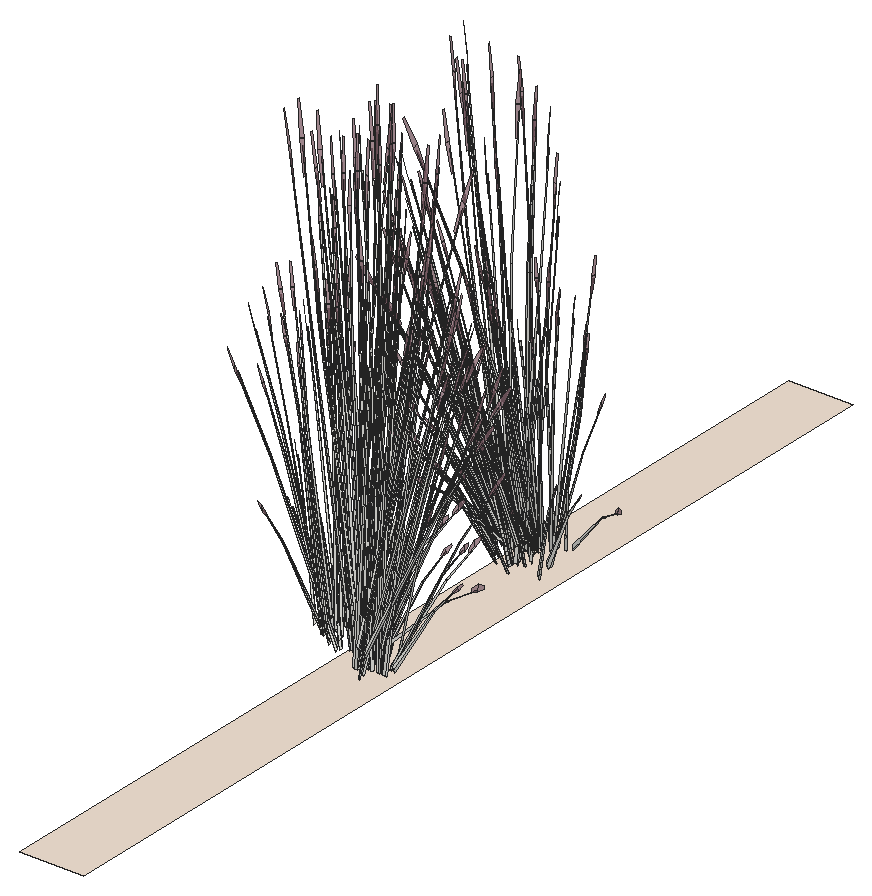
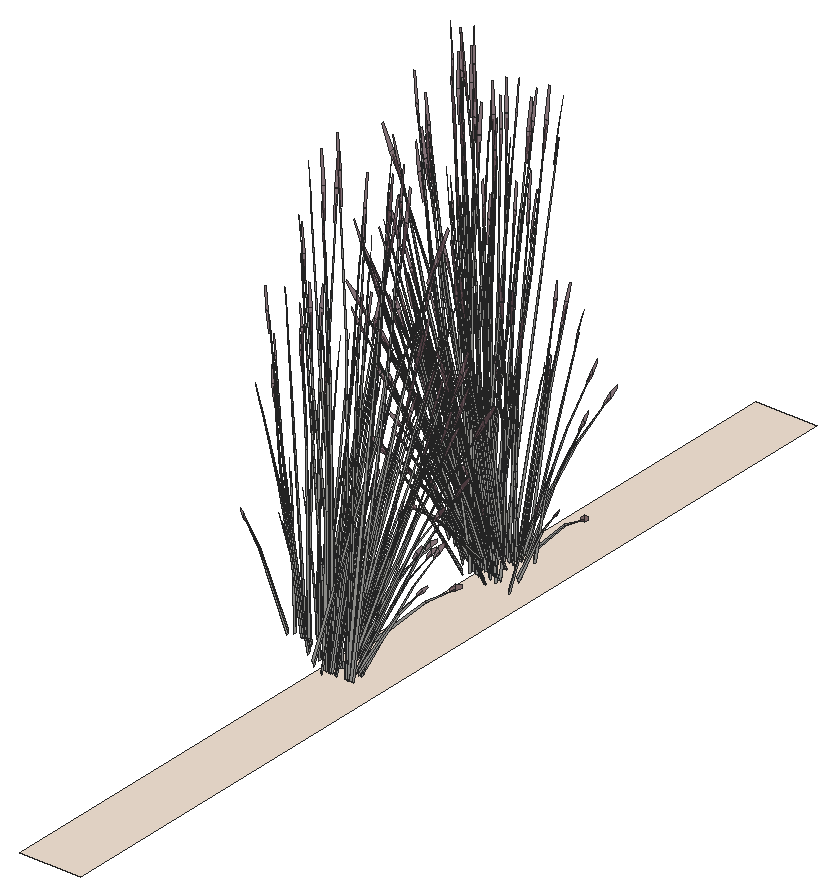
# SketchUp Ruby script. Lengths in inches.
U = 1.inch
M = Sketchup.active_model
def pt(a) = Geom::Point3d.new(a.map { |v| v * U })
def face(e, loops, mat)
  f = e.add_face(loops[0].map { |a| pt(a) })
  loops[1..].each { |l| e.add_face(l.map { |a| pt(a) }).erase! }
  f.material = f.back_material = mat if mat
  f
end
# faces: each face lists its corners as indices into pts; further lists are holes
def faces(e, pts, list, mat = nil) = list.each { |f| face(e, (f[0].is_a?(Array) ? f : [f]).map { |l| l.map { |i| pts[i] } }, mat) }
# xy, xz, yz: faces in a plane at the given z, y or x. An outline is a flat list of corners, or four numbers for a rectangle; further outlines are holes
def ring(l) = l.size == 4 ? [[l[0], l[1]], [l[2], l[1]], [l[2], l[3]], [l[0], l[3]]] : l.each_slice(2).to_a
def flat(e, list, mat, &to3) = list.each { |f| face(e, (f[0].is_a?(Array) ? f : [f]).map { |l| ring(l).map { |u, v| to3.(u, v) } }, mat) }
def xy(e, z, list, mat = nil) = flat(e, list, mat) { |x, y| [x, y, z] }
def xz(e, y, list, mat = nil) = flat(e, list, mat) { |x, z| [x, y, z] }
def yz(e, x, list, mat = nil) = flat(e, list, mat) { |y, z| [x, y, z] }
def lines(e, pts, list) = list.each { |a, b| e.add_line(pt(pts[a]), pt(pts[b])) }
# prism: a flat outline (further loops are holes) pulled along v
def prism(e, loops, v, mat = nil)
  f = face(e, loops, mat); d = Geom::Vector3d.new(v.map { |x| x * U })
  f.pushpull(f.normal.samedirection?(d) ? d.length : -d.length)
end
def box(e, o, s, mat = nil) = prism(e, [[o, [o[0] + s[0], o[1], o[2]], [o[0] + s[0], o[1] + s[1], o[2]], [o[0], o[1] + s[1], o[2]]]], [0, 0, s[2]], mat)
def at(x, y, z, deg = 0) = Geom::Transformation.translation(pt([x, y, z])) * Geom::Transformation.rotation(ORIGIN, Z_AXIS, deg.degrees)
def axes(o, x, y, z) = Geom::Transformation.new([*x, 0, *y, 0, *z, 0, *pt(o).to_a, 1])
def part(name) = M.definitions.add(name)
# library, detail: a bought-in or finely detailed component or shape, given as its bounding box
def library(name, o, s) = part(name).tap { |d| box(d.entities, o, s) }
def detail(e, o, s) = box(e.add_group.entities, o, s)
def put(e, d, t, mat = nil) = e.add_instance(d, t).tap { |i| i.material = mat if mat }
def group(e, t, mat = nil) = e.add_group.tap { |g| g.transformation = t; g.material = mat if mat }.entities
root = M.entities
M.materials.add("C01_Vanilla_Cream").color = [244, 228, 212]
M.materials.add("LightPink_Translucent").color = [144, 107, 117]
M.materials["LightPink_Translucent"].alpha = 0.75
c1 = part("blade")
p = [[2.15,0.21,22],[0,0.17,0],[0.09,0.45,0],[2.18,0.31,22],[2.29,0.31,22],[0.38,0.45,0],
  [2.48,0.24,33],[2.49,0.24,33],[2.48,0.22,33]]
faces(c1.entities,p,[[0,1,2,3],[4,5,2,3],[6,3,4,7],[8,0,3,6]])
c2 = part("seeds")
p = [[0.3,-0.1,1.38],[-0.01,-0.03,1.59],[-0.01,-0.03,0.03],[0.14,-0.07,-0.07],[0.29,-0.03,3],[0.15,0.01,3.11]]
faces(c2.entities,p,[[0,1,2,3],[1,0,4,5]],"LightPink_Translucent")
c3 = part("blade with seeds")
put(c3.entities,c1,at(0,0,0))
put(c3.entities,c2,axes([2.4,0.25,30.99],[1.5799,-0.05474,1.17369],[-0.12525,1.92788,0.29478],[-0.07173,-0.02425,1.56792]))
xy(root,48,[[354,216,360,306.76]],"C01_Vanilla_Cream")
put(root,c3,axes([358.93,250.65,50.91],[-0.23093,0.01116,1.28532],[0.15319,-0.4836,0.10393],[0.32909,0.02991,0.54946]))
put(root,c3,axes([359.23,249.6,49.52],[0.13078,0.42928,-0.23233],[-0.51941,0.1219,0.23233],[0.10471,0.0495,1.0423]))
put(root,c3,axes([360.13,251.32,51.55],[0.20448,0.33592,0.04823],[-0.37288,0.16442,0.37966],[0.16437,-0.03244,0.57892]))
put(root,c3,axes([358.1875,250.5625,49.79],[-0.70367,-0.1038,0.36899],[0.1432,-0.58624,0.1448],[0.10283,0.05661,1.2811]))
put(root,c3,axes([360.09,251.2,51.55],[-0.15729,0.44921,0.36002],[-0.51712,-0.15361,0.29685],[0.20336,-0.027,0.74497]))
put(root,c3,axes([357.625,252.01,49.65],[-0.18165,-0.42474,0],[0.51872,-0.14874,0],[0,0,1.15778]))
put(root,c3,axes([357.28,251.61,49.96],[-0.1074,0.43968,0.1086],[-0.52474,-0.07632,-0.3101],[-0.0955,-0.04515,0.95058]))
put(root,c3,axes([355.24,250.47,51.79],[0.46269,0.13744,0.2656],[-0.13495,0.40096,-0.3429],[-0.18628,0.03677,0.65611]))
put(root,c3,axes([358.31,251.95,49.64],[0.5845,-0.16716,-0.14398],[0.20539,0.48152,0.00006],[0.06452,-0.01848,1.30423]))
put(root,c3,axes([358.51,252.15,49.86],[0.16083,-0.48962,0.13232],[0.58854,0.13856,0.26315],[-0.10167,0.00238,1.20305]))
put(root,c3,axes([358.375,251.04,49.66],[0.38863,0.31822,0],[-0.38863,0.31822,0],[0,0,1.2695]))
put(root,c3,axes([356.17,250.44,50.51],[0.15825,-0.07127,1.32798],[0.05457,0.4976,0.10393],[-0.34278,0.06603,0.47463]))
put(root,c3,axes([359.43,250.9,49.86],[-0.43742,-0.35886,0.13232],[0.44081,-0.34807,0.26315],[-0.04831,0.07329,1.20305]))
put(root,c3,axes([358.62,250.36,49.54],[0.57914,0.08077,-0.46765],[-0.12221,0.49823,-0.12274],[0.17283,0.06037,1.03225]))
put(root,c3,axes([361.18,251.23,50.07],[-0.34399,0.08133,0.86145],[0.16192,-0.33614,0.63294],[0.18249,0.023,0.18974]))
put(root,c3,axes([357.5,252.2,49.65],[-0.56127,-0.22118,0],[0.27012,-0.45959,0],[0,0,1.2203]))
put(root,c3,axes([357.96,251.61,49.85],[-0.54364,-0.39653,-0.18894],[0.45745,-0.44527,0.41347],[-0.14639,0.04639,1.26162]))
put(root,c3,axes([356.53,252.375,49.86],[0.52105,0.24633,0.37238],[-0.31144,0.44171,0],[-0.11867,-0.0561,1.18128]))
put(root,c3,axes([358.37,250.67,50.04],[0.27012,-0.44393,0.33554],[0.56127,0.21365,-0.16149],[0,0.10233,1.07733]))
put(root,c3,axes([361.02,252.65,51.53],[-0.05034,-0.04313,1.33037],[0.11012,-0.46232,-0.12571],[0.1983,-0.02954,0.23543]))
put(root,c3,axes([354.47,250.78,51.54],[-0.09091,0.06396,1.31208],[0.00773,0.46734,-0.2075],[-0.20839,0.06078,0.10523]))
put(root,c3,axes([358.27,250.92,49.72],[0,0.56976,-0.04228],[-0.69617,0,0],[0,0.01791,1.34526]))
put(root,c3,axes([355.07,250.72,51.51],[-0.15083,0.44814,-0.38324],[-0.51712,-0.15361,-0.29685],[-0.2082,0.04109,0.7333]))
put(root,c3,axes([355.05,250.33,51.78],[0.28012,0.44611,-0.0912],[-0.49717,0.21923,-0.50621],[-0.20951,0.05886,0.76918]))
put(root,c3,axes([358.32,250.52,49.66],[0.33445,0.41351,-0.33554],[-0.50659,0.29119,0.16149],[0.10823,0.05117,1.07733]))
put(root,c3,axes([360.58,252.27,50.95],[-0.10656,-0.41414,-0.02619],[0.50364,-0.09521,-0.11874],[0.10517,0.02626,0.39164]))
put(root,c3,axes([356.23,252.63,49.78],[-0.34808,0.49367,0],[-0.58235,-0.27531,-0.38706],[-0.13264,-0.0627,1.22783]))
put(root,c3,axes([359.27,252.26,51.78],[0.02981,-0.50103,-0.0912],[0.56442,0.01369,-0.50621],[0.21738,0.0348,0.76918]))
put(root,c3,axes([359.79,250.92,49.86],[0,-0.49266,0.37238],[0.62289,0,0],[0,0.11221,1.18128]))
put(root,c3,axes([358.23,251.29,50.04],[0.60457,-0.03041,0.33554],[0.05467,0.50484,-0.16149],[-0.10823,0.05117,1.07733]))
put(root,c3,axes([358.6,250.77,49.96],[0.51872,-0.14368,0.1086],[0.18165,0.41027,-0.3101],[0,0.09029,0.95058]))
put(root,c3,axes([359.1875,252.06,51.79],[-0.31678,-0.30846,0.2656],[0.36171,-0.29199,-0.3429],[0.18378,0.04443,0.65611]))
put(root,c3,axes([357.6875,251.53,49.66],[-0.60457,0.03041,-0.33554],[-0.05467,-0.50484,0.16149],[-0.10823,0.05117,1.07733]))
put(root,c3,axes([360.53,251.77,49.94],[-0.13408,-0.12117,1.07251],[0.17446,-0.40083,-0.23066],[0.27128,0.0543,0.45856]))
put(root,c3,axes([358.14,252.21,49.65],[0.56127,0.22118,0],[-0.27012,0.45959,0],[0,0,1.31215]))
put(root,c3,axes([359.76,251.95,51.54],[0.11943,-0.00833,1.31208],[0.32759,-0.38275,-0.2075],[0.21244,0.05052,0.10523]))
put(root,c3,axes([358.36,252.7,49.64],[-0.34375,-0.4954,-0.03857],[0.58235,-0.27531,0.38706],[-0.1435,0.04717,1.22723]))
put(root,c3,axes([358.24,251.5,49.96],[0.41131,0.296,0.1086],[-0.34309,0.33395,-0.3101],[-0.0955,0.04515,0.95058]))
put(root,c3,axes([354.99,251.58,51.55],[-0.13808,-0.45342,0.36002],[0.54163,-0.07869,0.29685],[-0.15963,0.10664,0.74497]))
put(root,c3,axes([354.88,251.49,51.55],[-0.3822,-0.20719,0.04823],[0.22252,-0.29505,0.37966],[-0.12254,0.09539,0.57892]))
put(root,c3,axes([355.06,250.95,50.91],[0.19317,-0.10421,1.28532],[0.16263,0.48153,0.10393],[-0.30326,0.10883,0.54946]))
put(root,c3,axes([359.3,252.01,51.74],[0.55654,0.01186,-0.53284],[-0.03738,0.49951,0.0643],[0.23578,0.05271,0.75375]))
put(root,c3,axes([358.67,252.41,49.86],[0.52105,-0.24633,0.37238],[0.31144,0.44171,0],[-0.11867,0.0561,1.18128]))
put(root,c3,axes([357.93,252.03,49.72],[0.24206,0.56598,-0.04509],[-0.69162,0.19832,0],[0.00845,0.01976,1.2913]))
put(root,c3,axes([358.2,252.64,49.52],[-0.51941,-0.1219,-0.23233],[0.13078,-0.42928,0.23233],[-0.10471,0.0495,1.0423]))
put(root,c3,axes([354.45,251.77,49.94],[0.19348,0.04044,1.07251],[0.1247,0.41309,-0.23066],[-0.26282,0.07733,0.45856]))
put(root,c3,axes([355.32,251.43,51.79],[0.48462,-0.07041,0.2656],[0.12797,0.4025,-0.3429],[-0.13888,0.10811,0.65611]))
put(root,c3,axes([360.21,251,49.78],[0.69617,0,0],[0,0.55062,-0.38706],[0,0.12541,1.22783]))
put(root,c3,axes([353.46,251.25,51.53],[0.07105,0.01321,1.33037],[0.2198,0.43529,-0.12571],[-0.14545,0.11425,0.23543]))
put(root,c3,axes([359.93,251.28,49.65],[-0.69582,-0.00394,-0.03732],[0,-0.55062,0.37457],[-0.02187,0.12535,1.18764]))
put(root,c3,axes([358.43,250.8,50],[0.62699,0.23507,-0.21822],[-0.3019,0.49615,-0.37502],[0.0197,0.12182,1.19781]))
put(root,c3,axes([354.05,252.63,50.07],[0.23202,-0.22328,0.86145],[0.09155,0.35348,0.63294],[-0.16768,0.06329,0.18974]))
put(root,c3,axes([359.64,252.22,51.39],[0.31678,0.30846,-0.2656],[-0.36171,0.29199,0.3429],[0.18378,0.04443,0.65611]))
put(root,c3,axes([359.79,251.36,49.52],[-0.38863,0.30738,-0.23233],[-0.38863,-0.30738,0.23233],[0,0.09901,1.0423]))
put(root,c3,axes([358.11,251.39,50],[0.06488,0.56215,-0.21822],[-0.6757,0.03399,-0.37502],[-0.11898,0.07488,1.19781]))
put(root,c3,axes([359.47,252.34,51.55],[-0.02803,0.37463,0.04823],[-0.42332,-0.01027,0.37966],[0.16216,0.0392,0.57892]))
put(root,c3,axes([358.36,251.17,49.66],[-0.27012,0.44393,-0.33554],[-0.56127,-0.21365,0.16149],[0,0.10233,1.07733]))
put(root,c3,axes([354.93,251.67,51.39],[-0.48462,0.07041,-0.2656],[-0.12797,-0.4025,0.3429],[-0.13888,0.10811,0.65611]))
put(root,c3,axes([359.51,252.22,51.55],[-0.41051,0.32462,0.36002],[-0.35404,-0.34474,0.29685],[0.1926,0.05988,0.74497]))
put(root,c3,axes([354.22,252.57,52.23],[0.49129,0.13151,-0.04866],[-0.15113,0.40475,-0.22062],[-0.08035,0.06145,0.72768]))
put(root,c3,axes([357.71,251.82,49.54],[-0.375,0.3703,-0.46765],[-0.46584,-0.33578,-0.12274],[-0.15027,0.09237,1.03225]))
put(root,c3,axes([358.21,252.59,51.79],[-0.08599,-0.39682,0.2656],[0.49155,-0.10478,-0.3429],[0.13203,0.11372,0.65611]))
put(root,c3,axes([358.375,252.45,49.75],[0.697,0.16013,0.23067],[-0.17437,0.57237,-0.27369],[-0.11536,0.07164,1.23664]))
put(root,c3,axes([358.32,252.83,49.51],[-0.52105,0.24633,-0.37238],[-0.31144,-0.44171,0],[-0.11867,0.0561,1.18128]))
put(root,c3,axes([360.06,251.375,49.51],[0,0.49266,-0.37238],[-0.62289,0,0],[0,0.11221,1.18128]))
put(root,c3,axes([358.5,251.43,50.91],[-0.2068,-0.08488,1.28532],[0.42797,-0.35609,0.10393],[0.26673,0.16064,0.54946]))
put(root,c3,axes([358.54,250.3125,51.36],[-0.48108,-0.25598,1.03712],[0.50798,-0.39855,0.44749],[0.15521,0.24018,1.00248]))
put(root,c3,axes([355.07,251.39,51.78],[0.515,0.27165,-0.0912],[-0.2967,0.3934,-0.50621],[-0.1455,0.13675,0.76918]))
put(root,c3,axes([359.26,252.4,50.07],[-0.31347,-0.14166,0.86145],[0.40476,-0.14393,0.63294],[0.10917,0.12192,0.18974]))
put(root,c3,axes([358.16,252.8,51.78],[0.33176,-0.4217,-0.0912],[0.48044,0.24295,-0.50621],[0.16701,0.11914,0.76918]))
put(root,c3,axes([355.76,251.27,50.91],[0.13906,-0.15138,1.28532],[0.35111,0.40859,0.10393],[-0.24082,0.18608,0.54946]))
put(root,c3,axes([355.33,251.71,51.51],[0.14302,0.44985,-0.38324],[-0.54163,0.07869,-0.29685],[-0.15522,0.12083,0.7333]))
put(root,c3,axes([355.98,252.23,51.79],[0.3767,-0.25939,0.2656],[0.3566,0.29618,-0.3429],[-0.05426,0.15048,0.65611]))
put(root,c3,axes([358.8,252.76,49.78],[0.34808,0.49367,0],[-0.58235,0.27531,-0.38706],[-0.13264,0.0627,1.22783]))
put(root,c3,axes([357.73,253.15,51.53],[0.00165,-0.05965,1.33037],[0.47711,-0.26315,-0.12571],[0.16572,0.09393,0.23543]))
put(root,c3,axes([359.35,252.92,49.12],[0.04056,-0.07113,1.32257],[0.51066,-0.20948,-0.20205],[0.15482,0.10842,0.22528]))
put(root,c3,axes([358.5,250.8,50.13],[-0.01521,-0.46386,1.05954],[0.68831,0.12024,0.44862],[-0.1628,0.25382,1.00012]))
put(root,c3,axes([358.68,251.31,49.57],[0.20414,0.45107,-0.51909],[-0.58805,0.16245,-0.13624],[0.02256,0.15274,1.1458]))
put(root,c3,axes([355.63,252.47,51.55],[-0.45752,-0.02296,0.04823],[0.01254,-0.34663,0.37966],[-0.04787,0.13278,0.57892]))
put(root,c3,axes([354.66,252.86,49.12],[0.07468,0.04922,1.32257],[0.12663,0.45605,-0.20205],[-0.16551,0.09725,0.22528]))
put(root,c3,axes([355.78,252.5,51.55],[-0.39645,-0.33614,0.36002],[0.42102,-0.2899,0.29685],[-0.07313,0.15771,0.74497]))
put(root,c3,axes([358.56,252.59,51.51],[0.54938,-0.11711,-0.38324],[0.0961,0.44351,-0.29685],[0.14756,0.1271,0.7333]))
put(root,c3,axes([357.03,252.66,51.79],[0.16784,-0.37886,0.2656],[0.48968,0.1105,-0.3429],[0.0449,0.15254,0.65611]))
put(root,c3,axes([359.3125,253.04,50],[-0.35702,-0.01545,0.78795],[0.23577,-0.32816,0.43504],[0.14104,0.11659,0.61808]))
put(root,c3,axes([358.29,252.95,51.55],[-0.25304,0.31296,0.04823],[-0.36033,-0.18221,0.37966],[0.11649,0.10034,0.57892]))
put(root,c3,axes([357.69,254.01,52.23],[0.38473,-0.28263,-0.04866],[0.35252,0.30954,-0.22062],[0.02482,0.08771,0.72768]))
put(root,c3,axes([358.39,252.87,51.55],[-0.55374,0.11306,0.36002],[-0.0961,-0.44351,0.29685],[0.13023,0.13071,0.74497]))
put(root,c3,axes([355.66,251.64,50.91],[0.10366,-0.16934,1.28532],[0.43488,0.35044,0.10393],[-0.19618,0.21841,0.54946]))
put(root,c3,axes([358.15,252.24,49.94],[0.00982,-0.16331,1.07251],[0.4695,-0.18242,-0.23066],[0.14493,0.19547,0.45856]))
put(root,c3,axes([356.88,253,51.55],[-0.41024,0.16744,0.04823],[-0.2008,-0.30532,0.37966],[0.03962,0.13459,0.57892]))
put(root,c3,axes([355.78,252.6,51.39],[-0.3767,0.25939,-0.2656],[-0.3566,-0.29618,0.3429],[-0.05426,0.15048,0.65611]))
put(root,c3,axes([354.48,252.52,51.54],[-0.01384,0.09749,1.31208],[0.39274,0.33916,-0.2075],[-0.10282,0.16039,0.10523]))
put(root,c3,axes([355.74,252.3,52.05],[0.61188,0.02441,-0.10123],[-0.01672,0.46217,-0.56189],[-0.0425,0.178,0.85379]))
put(root,c3,axes([356.87,252.82,51.78],[0.54481,-0.22937,-0.0912],[0.26773,0.4071,-0.50621],[0.07188,0.17155,0.76918]))
put(root,c3,axes([357.03,252.97,51.8],[-0.54859,-0.1288,0.39962],[0.18759,-0.42344,0.32951],[0.03297,0.16652,0.82692]))
put(root,c3,axes([356.02,253.61,50.07],[-0.01441,-0.29294,0.86145],[0.36003,0.20894,0.63294],[-0.07081,0.13963,0.18974]))
put(root,c3,axes([356.97,252.91,49.12],[0.0901,-0.02681,1.32257],[0.54199,0.14755,-0.20205],[0.01585,0.1663,0.22528]))
put(root,c3,axes([356.15,252.48,51.75],[0.39855,0.33102,-0.4254],[-0.42102,0.2899,-0.32951],[-0.06064,0.16819,0.81396]))
put(root,c3,axes([355.72,252.97,50.12],[0.50577,-0.08724,0.04881],[0.11627,0.35148,-0.64728],[-0.03206,0.17792,0.5802]))
put(root,c3,axes([357.34,252.8,51.51],[0.54728,0.1235,-0.38324],[-0.18759,0.42344,-0.29685],[0.05018,0.17048,0.7333]))
put(root,c3,axes([357.65,251.92,50.91],[-0.12726,-0.15818,1.28532],[0.58807,-0.13317,0.10393],[0.13291,0.24832,0.54946]))
put(root,c3,axes([357.09,253.06,51.39],[-0.16784,0.37886,-0.2656],[-0.48968,-0.1105,0.3429],[0.0449,0.15254,0.65611]))
put(root,c3,axes([356.03,252.32,52],[-0.01449,0.45571,-0.59145],[-0.61002,-0.03061,0.07138],[-0.06438,0.19306,0.83667]))
put(root,c3,axes([354.4375,253.52,51.53],[0.06316,-0.02974,1.33037],[0.52204,0.19785,-0.12571],[-0.01227,0.16473,0.23543]))
put(root,c3,axes([356.61,252,50.91],[-0.01363,-0.18909,1.28532],[0.5906,0.12544,0.10393],[-0.03653,0.26947,0.54946]))
put(root,c3,axes([357.14,252.72,51.74],[0.26572,0.40059,-0.53284],[-0.54698,0.22325,0.0643],[0.06214,0.19355,0.75375]))
put(root,c3,axes([355.6,253.35,49.94],[0.17569,-0.07772,1.07251],[0.43377,0.23434,-0.23066],[-0.12911,0.20277,0.45856]))
put(root,c3,axes([356.74,253.73,51.54],[0.07057,0.07933,1.31208],[0.56952,0.03117,-0.2075],[0.05727,0.17496,0.10523]))
put(root,c3,axes([355.83,252.97,50.52],[0.01223,-0.25433,1.15759],[0.55017,0.13434,0.15997],[-0.04767,0.27105,0.54661]))
put(root,c3,axes([356.25,270.38,50.91],[0.12726,0.15818,1.28532],[-0.58807,0.13317,0.10393],[-0.13291,-0.24832,0.54946]))
put(root,c3,axes([357.22,269.33,51.54],[-0.08515,-0.06907,1.31208],[-0.56828,0.04379,-0.2075],[-0.0907,-0.16522,0.10523]))
put(root,c3,axes([358.54,270.15,49.94],[-0.15825,0.09972,1.07251],[-0.47395,-0.17454,-0.23066],[0.08785,-0.21706,0.45856]))
put(root,c3,axes([357.82,270.5,51.74],[-0.26572,-0.40059,-0.53284],[0.54698,-0.22325,0.0643],[-0.06214,-0.19355,0.75375]))
put(root,c3,axes([356.09,269.96,49.94],[-0.03371,0.16116,1.07251],[-0.49286,0.13491,-0.23066],[-0.11521,-0.20831,0.45856]))
put(root,c3,axes([357.36,269.61,49.12],[-0.09338,0.01775,1.32257],[-0.51641,-0.1998,-0.20205],[0.00867,-0.16666,0.22528]))
put(root,c3,axes([358.92,270.89,51.74],[0.01449,-0.45571,-0.53284],[0.61002,0.03061,0.0643],[0.06438,-0.19306,0.75375]))
put(root,c3,axes([359.77,270.18,51.54],[-0.00537,-0.09805,1.31208],[-0.45391,-0.28338,-0.2075],[0.07018,-0.17178,0.10523]))
put(root,c3,axes([357.87,270.16,51.39],[0.16784,-0.37886,-0.2656],[0.48968,0.1105,0.3429],[-0.0449,-0.15254,0.65611]))
put(root,c3,axes([358.24,270.66,50.91],[-0.10366,0.16934,1.28532],[-0.43488,-0.35044,0.10393],[0.19618,-0.21841,0.54946]))
put(root,c3,axes([359.65,269.82,51.53],[-0.05654,0.03763,1.33037],[-0.55396,-0.12696,-0.12571],[-0.02005,-0.16422,0.23543]))
put(root,c3,axes([357.62,270.42,51.51],[-0.54728,-0.1235,-0.38324],[0.18759,-0.42344,-0.29685],[-0.05018,-0.17048,0.7333]))
put(root,c3,axes([357.95,269.36,50.07],[0.07142,0.28728,0.86145],[-0.3962,-0.15911,0.63294],[0.04263,-0.1471,0.18974]))
put(root,c3,axes([358.8,270.74,51.51],[-0.39855,-0.33102,-0.38324],[0.42102,-0.2899,-0.29685],[0.06064,-0.16819,0.7333]))
put(root,c3,axes([356.64,269.1,51.53],[-0.01039,0.05905,1.33037],[-0.51226,0.21431,-0.12571],[-0.15074,-0.10955,0.23543]))
put(root,c3,axes([356.52,270.15,51.82],[0.62019,-0.12663,0.40322],[0.10763,0.49673,0.33247],[-0.14586,-0.1464,0.83437]))
put(root,c3,axes([357.93,270.24,51.55],[0.54859,0.1288,0.36002],[-0.18759,0.42344,0.29685],[-0.03297,-0.16652,0.74497]))
put(root,c3,axes([358.08,270.4,51.78],[-0.54481,0.22937,-0.0912],[-0.26773,-0.4071,-0.50621],[-0.07188,-0.17155,0.76918]))
put(root,c3,axes([359.22,270.91,51.78],[-0.61188,-0.02441,-0.0912],[0.01672,-0.46217,-0.50621],[0.0425,-0.178,0.76918]))
put(root,c3,axes([359.17,270.61,51.39],[0.3767,-0.25939,-0.2656],[0.3566,0.29618,0.3429],[0.05426,-0.15048,0.65611]))
put(root,c3,axes([355.92,269.7,50.07],[0.29042,0.17147,0.86145],[-0.42295,0.10307,0.63294],[-0.0905,-0.13178,0.18974]))
put(root,c3,axes([358.07,270.21,51.55],[0.41024,-0.16744,0.04823],[0.2008,0.30532,0.37966],[-0.03962,-0.13459,0.57892]))
put(root,c3,axes([356.62,270.61,51.74],[-0.47473,-0.23813,-0.53284],[0.33738,-0.41728,0.0643],[-0.172,-0.14218,0.75375]))
put(root,c3,axes([356.45,270.29,51.39],[-0.08599,-0.39682,-0.2656],[0.49155,-0.10478,0.3429],[-0.13203,-0.11372,0.65611]))
put(root,c3,axes([356.67,270.26,51.55],[0.25304,-0.31296,0.04823],[0.36033,0.18221,0.37966],[-0.11649,-0.10034,0.57892]))
put(root,c3,axes([355.6875,270.22,49.12],[-0.05393,0.0649,1.32257],[-0.545,0.13993,-0.20205],[-0.13166,-0.12729,0.22528]))
put(root,c3,axes([356.59,272,49.57],[-0.22864,-0.5052,-0.52377],[0.65862,-0.18195,-0.13747],[-0.02527,-0.17107,1.15612]))
put(root,c3,axes([355.4,270.87,50.91],[0.2068,0.08488,1.28532],[-0.42797,0.35609,0.10393],[-0.26673,-0.16064,0.54946]))
put(root,c3,axes([359.64,270.46,49.12],[-0.08333,-0.03881,1.32257],[-0.21404,-0.4336,-0.20205],[0.14439,-0.11767,0.22528]))
put(root,c3,axes([357.92,270.55,51.79],[-0.16784,0.37886,0.2656],[-0.48968,-0.1105,-0.3429],[-0.0449,-0.15254,0.65611]))
put(root,c3,axes([356.4,270.62,51.51],[-0.54938,0.11711,-0.38324],[-0.0961,-0.44351,-0.29685],[-0.14756,-0.1271,0.7333]))
put(root,c3,axes([359.17,270.71,51.55],[0.39645,0.33614,0.36002],[-0.42102,0.2899,0.29685],[0.07313,-0.15771,0.74497]))
put(root,c3,axes([356.78,270.23,52.07],[-0.37157,0.4723,-0.10215],[-0.5381,-0.2721,-0.56695],[-0.18705,-0.13344,0.86148]))
put(root,c3,axes([359.32,270.75,51.55],[0.45752,0.02296,0.04823],[-0.01254,0.34663,0.37966],[0.04787,-0.13278,0.57892]))
put(root,c3,axes([358.98,270.98,51.79],[-0.3767,0.25939,0.2656],[-0.3566,-0.29618,-0.3429],[0.05426,-0.15048,0.65611]))
put(root,c3,axes([359.64,271.68,51.74],[0.29081,-0.38873,-0.53284],[0.5096,0.27626,0.0643],[0.17364,-0.14084,0.75375]))
put(root,c3,axes([356.5,270.55,49.78],[-0.34808,-0.49367,0],[0.58235,-0.27531,-0.38706],[0.13264,-0.0627,1.22783]))
put(root,c3,axes([359.625,271.5,51.51],[-0.14302,-0.44985,-0.38324],[0.54163,-0.07869,-0.29685],[0.15522,-0.12083,0.7333]))
put(root,c3,axes([357.26,269.95,49.6],[-0.38473,0.28263,-0.02919],[-0.35252,-0.30954,-0.13237],[-0.02482,-0.08771,0.43661]))
put(root,c3,axes([355.36,270.09,51.54],[-0.11979,-0.00348,1.31208],[-0.38137,0.34775,-0.2075],[-0.20349,-0.07106,0.10523]))
put(root,c3,axes([359.88,271.82,51.78],[-0.515,-0.27165,-0.0912],[0.2967,-0.3934,-0.50621],[0.1455,-0.13675,0.76918]))
put(root,c3,axes([357.75,273.3,50.49],[0.48111,0.19866,1.13446],[-0.47133,0.42798,0.44862],[-0.21112,-0.25366,0.95105]))
put(root,c3,axes([356.75,270.62,51.79],[0.08599,0.39682,0.2656],[-0.49155,0.10478,-0.3429],[-0.13203,-0.11372,0.65611]))
put(root,c3,axes([355.24,271.93,49.51],[0,-0.49266,-0.37238],[0.62289,0,0],[0,-0.11221,1.18128]))
put(root,c3,axes([356.97,270.47,49.51],[0.52105,-0.24633,-0.37238],[0.31144,0.44171,0],[0.11867,-0.0561,1.18128]))
put(root,c3,axes([360.0625,271.32,49.94],[-0.19889,-0.01459,1.07251],[-0.20376,-0.39145,-0.23066],[0.24434,-0.11074,0.45856]))
put(root,c3,axes([355.27,270.875,51.82],[0.45978,-0.36358,0.40322],[0.39653,0.38611,0.33247],[-0.21571,-0.06707,0.83437]))
put(root,c3,axes([361.15,271.7,51.53],[-0.07272,-0.00374,1.33037],[-0.30197,-0.40092,-0.12571],[0.12127,-0.13182,0.23543]))
put(root,c3,axes([357.59,271.48,49.54],[0.375,-0.3703,-0.46765],[0.46584,0.33578,-0.12274],[0.15027,-0.09237,1.03225]))
put(root,c3,axes([360.29,270.6,50.07],[-0.18544,0.25079,0.86145],[-0.15939,-0.33694,0.63294],[0.15316,-0.08443,0.18974]))
put(root,c3,axes([360.03,271.55,51.39],[0.48462,-0.07041,-0.2656],[0.12797,0.4025,0.3429],[0.13888,-0.10811,0.65611]))
put(root,c3,axes([355.48,270.875,51.55],[0.02803,-0.37463,0.04823],[0.42332,0.01027,0.37966],[-0.16216,-0.0392,0.57892]))
put(root,c3,axes([356.93,272.13,49.66],[0.27012,-0.44393,-0.33554],[0.56127,0.21365,0.16149],[0,-0.10233,1.07733]))
put(root,c3,axes([355.32,270.99,51.39],[-0.31678,-0.30846,-0.2656],[0.36171,-0.29199,0.3429],[-0.18378,-0.04443,0.65611]))
put(root,c3,axes([357.18,271.91,50],[-0.06488,-0.56215,-0.21822],[0.6757,-0.03399,-0.37502],[0.11898,-0.07488,1.19781]))
put(root,c3,axes([355.51,271.94,49.52],[0.38863,-0.30738,-0.23233],[0.38863,0.30738,0.23233],[0,-0.09901,1.0423]))
put(root,c3,axes([355.35,270.47,49.6],[-0.1606,0.40228,-0.02919],[-0.4943,-0.12375,-0.13237],[-0.07505,-0.0658,0.43661]))
put(root,c3,axes([359.63,271.78,51.79],[-0.48462,0.07041,0.2656],[-0.12797,-0.4025,-0.3429],[0.13888,-0.10811,0.65611]))
put(root,c3,axes([356.87,272.5,50],[-0.62699,-0.23507,-0.21822],[0.3019,-0.49615,-0.37502],[-0.0197,-0.12182,1.19781]))
put(root,c3,axes([355.08,272.3,49.78],[-0.69617,0,0],[0,-0.55062,-0.38706],[0,-0.12541,1.22783]))
put(root,c3,axes([355.2,271.32,49.94],[0.1087,0.13716,1.07251],[-0.25048,0.37284,-0.23066],[-0.25719,-0.08912,0.45856]))
put(root,c3,axes([357.09,270.67,49.52],[0.51941,0.1219,-0.23233],[-0.13078,0.42928,0.23233],[0.10471,-0.0495,1.0423]))
put(root,c3,axes([355.65,271.2,51.74],[-0.55654,-0.01186,-0.53284],[0.03738,-0.49951,0.0643],[-0.23578,-0.05271,0.75375]))
put(root,c3,axes([360.07,271.72,51.55],[0.3822,0.20719,0.04823],[-0.22252,0.29505,0.37966],[0.12254,-0.09539,0.57892]))
put(root,c3,axes([359.96,271.63,51.55],[0.13808,0.45342,0.36002],[-0.54163,0.07869,0.29685],[0.15963,-0.10664,0.74497]))
put(root,c3,axes([361.42,272.18,51.54],[0.07726,-0.07504,1.31208],[-0.09888,-0.46032,-0.2075],[0.19384,-0.08728,0.10523]))
put(root,c3,axes([355.625,272.16,49.75],[-0.51786,0.4142,0.23067],[-0.51817,-0.40984,-0.27369],[-0.01808,-0.11762,1.23664]))
put(root,c3,axes([354.9,270.38,51.53],[0.04127,0.04917,1.33037],[-0.19898,0.44196,-0.12571],[-0.20151,0.0032,0.23543]))
put(root,c3,axes([357.27,272.35,49.82],[0.6273,0.23878,0.18048],[-0.3019,0.49615,0.37502],[0,-0.11437,1.20407]))
put(root,c3,axes([357.03,273.02,49.83],[0.14756,-0.58378,-0.17572],[0.69966,0.10176,0.38453],[-0.12225,-0.08062,1.1733]))
put(root,c3,axes([355.47,271.3,51.51],[-0.40426,0.32635,-0.38324],[-0.35404,-0.34474,-0.29685],[-0.2054,-0.04965,0.7333]))
put(root,c3,axes([355.77,271.15,51.79],[0.31678,0.30846,0.2656],[-0.36171,0.29199,-0.3429],[-0.18378,-0.04443,0.65611]))
put(root,c3,axes([354.56,271.73,50.07],[0.35544,-0.03525,0.86145],[-0.22547,0.31061,0.63294],[-0.17565,-0.04659,0.18974]))
put(root,c3,axes([357.07,272.02,50.04],[-0.60457,0.03041,0.33554],[-0.05467,-0.50484,-0.16149],[0.10823,-0.05117,1.07733]))
put(root,c3,axes([355.68,270.96,51.78],[-0.02981,0.50103,-0.0912],[-0.56442,-0.01369,-0.50621],[-0.21738,-0.0348,0.76918]))
put(root,c3,axes([355.51,272.39,49.86],[0,0.49266,0.37238],[-0.62289,0,0],[0,-0.11221,1.18128]))
